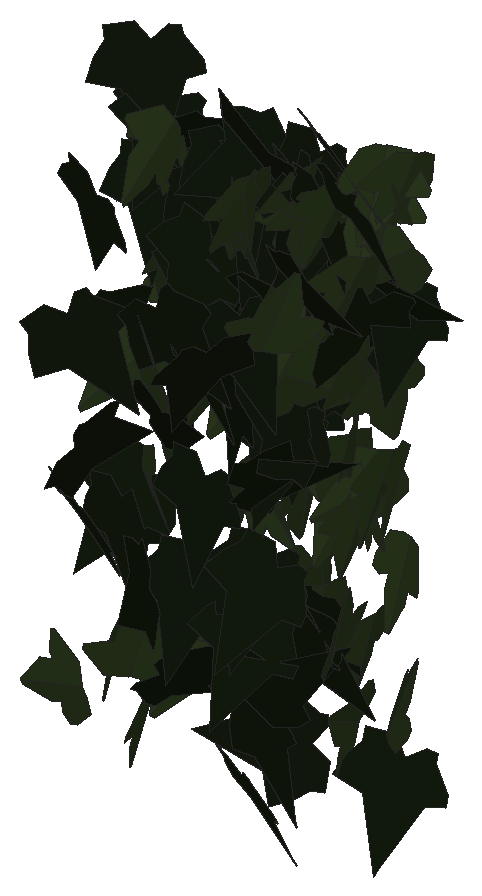
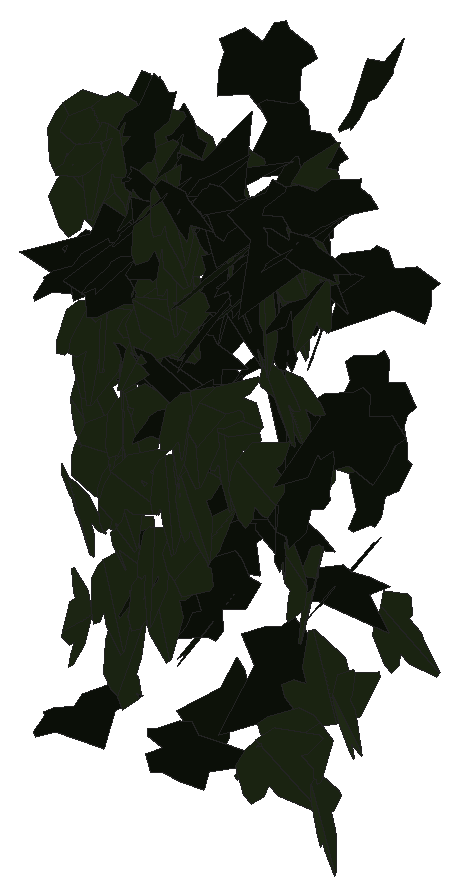
# SketchUp Ruby script. Lengths in inches.
U = 1.inch
M = Sketchup.active_model
def pt(a) = Geom::Point3d.new(a.map { |v| v * U })
def face(e, loops, mat)
  f = e.add_face(loops[0].map { |a| pt(a) })
  loops[1..].each { |l| e.add_face(l.map { |a| pt(a) }).erase! }
  f.material = f.back_material = mat if mat
  f
end
# faces: each face lists its corners as indices into pts; further lists are holes
def faces(e, pts, list, mat = nil) = list.each { |f| face(e, (f[0].is_a?(Array) ? f : [f]).map { |l| l.map { |i| pts[i] } }, mat) }
# xy, xz, yz: faces in a plane at the given z, y or x. An outline is a flat list of corners, or four numbers for a rectangle; further outlines are holes
def ring(l) = l.size == 4 ? [[l[0], l[1]], [l[2], l[1]], [l[2], l[3]], [l[0], l[3]]] : l.each_slice(2).to_a
def flat(e, list, mat, &to3) = list.each { |f| face(e, (f[0].is_a?(Array) ? f : [f]).map { |l| ring(l).map { |u, v| to3.(u, v) } }, mat) }
def xy(e, z, list, mat = nil) = flat(e, list, mat) { |x, y| [x, y, z] }
def xz(e, y, list, mat = nil) = flat(e, list, mat) { |x, z| [x, y, z] }
def yz(e, x, list, mat = nil) = flat(e, list, mat) { |y, z| [x, y, z] }
def lines(e, pts, list) = list.each { |a, b| e.add_line(pt(pts[a]), pt(pts[b])) }
# prism: a flat outline (further loops are holes) pulled along v
def prism(e, loops, v, mat = nil)
  f = face(e, loops, mat); d = Geom::Vector3d.new(v.map { |x| x * U })
  f.pushpull(f.normal.samedirection?(d) ? d.length : -d.length)
end
def box(e, o, s, mat = nil) = prism(e, [[o, [o[0] + s[0], o[1], o[2]], [o[0] + s[0], o[1] + s[1], o[2]], [o[0], o[1] + s[1], o[2]]]], [0, 0, s[2]], mat)
def at(x, y, z, deg = 0) = Geom::Transformation.translation(pt([x, y, z])) * Geom::Transformation.rotation(ORIGIN, Z_AXIS, deg.degrees)
def axes(o, x, y, z) = Geom::Transformation.new([*x, 0, *y, 0, *z, 0, *pt(o).to_a, 1])
def part(name) = M.definitions.add(name)
# library, detail: a bought-in or finely detailed component or shape, given as its bounding box
def library(name, o, s) = part(name).tap { |d| box(d.entities, o, s) }
def detail(e, o, s) = box(e.add_group.entities, o, s)
def put(e, d, t, mat = nil) = e.add_instance(d, t).tap { |i| i.material = mat if mat }
def group(e, t, mat = nil) = e.add_group.tap { |g| g.transformation = t; g.material = mat if mat }.entities
root = M.entities
M.materials.add("efeu1").color = [18, 25, 13]
M.materials.add("efeu2").color = [43, 57, 29]
c1 = part("ivyleaf_9")
p = [[1.54,2.16,1.25],[1.36,2.04,1.19],[-0.21,0.99,0.68],[-0.71,1.11,0.82],[-0.85,0.86,0.67],[-0.8,0.17,0.21],
  [-0.9,-0.01,0.1],[-0.67,-0.16,-0.02],[-0.08,-0.08,-0.05],[-0.03,-0.6,-0.4],[0.65,-0.88,-0.66],[0.83,-0.6,-0.49],
  [1.29,-0.42,-0.43],[1.8125,-0.07,-0.26],[1.21,0.44,0.15]]
faces(c1.entities,p,[[0,1,2,3,4,5,6,7,8,9,10,11,12,13,14]],"efeu1")
c2 = part("ivyleaf_10")
p = [[0,0.5,-0.03],[-0.0625,2.02,-0.43],[-0.19,2.01,-0.46],[-0.54,1.05,-0.29],[-0.52,0.625,-0.18],[-0.83,0.76,-0.28],
  [-1.16,0.64,-0.33],[-1.15,0.33,-0.24],[-0.77,-0.39,0.02],[-0.3,-0.51,0.16],[0.04,-0.48,0.23],[-0.02,2.01,-0.4375],
  [-0.06,2.01,-0.43],[0.04,-0.49,0.23],[0.67,-0.49,0.14],[1.38,0.36,-0.2],[1.375,0.51,-0.24],[0.81,0.65,-0.19],
  [0.62,0.59,-0.15],[0.6,1.09,-0.28],[0.5,1.23,-0.31]]
faces(c2.entities,p,[[0,1,2,3,4,5,6,7,8,9,10],[11,12,0,13,14,15,16,17,18,19,20]],"efeu2")
put(root,c1,axes([14.76,220.19,218.36],[0.00233,-0.19291,0.46128],[-0.0176,-0.46103,-0.19272],[0.49968,-0.01534,-0.00894]))
put(root,c1,axes([15.89,219.92,222.17],[-0.00179,0.43095,-0.25353],[0.00643,-0.25349,-0.43093],[-0.49996,-0.0048,-0.00464]))
put(root,c1,axes([13.15,221.18,222.89],[0.04405,-0.3663,0.33747],[0.11155,-0.32293,-0.36507],[0.4854,0.10745,0.05327]))
put(root,c2,axes([14.5,220.78,220.76],[-0.34497,0.29007,-0.21646],[-0.16391,0.1414,0.45071],[0.32269,0.38192,-0.00247]))
put(root,c1,axes([14.4,220.875,221.83],[-0.09481,-0.07375,-0.48536],[0.36921,0.31509,-0.12],[0.32356,-0.38115,-0.00529]))
put(root,c1,axes([14.35,221.52,221.02],[0.26151,-0.37801,0.19676],[0.11597,-0.15902,-0.45963],[0.41008,0.28604,0.0045]))
put(root,c1,axes([14.35,221.82,219.04],[0.01013,-0.48128,0.13516],[-0.00187,-0.13522,-0.48136],[0.49989,0.00925,-0.00454]))
put(root,c2,axes([12.44,221.62,215.58],[-0.14932,0.01669,0.47689],[-0.47701,-0.01868,-0.1487],[0.01285,-0.49937,0.0215]))
put(root,c1,axes([12.4375,221.58,220.76],[-0.09135,-0.19879,-0.4496],[0.23418,0.38447,-0.21758],[0.43222,-0.25032,0.02286]))
put(root,c1,axes([12.17,222.09,217.77],[0.16583,-0.32378,0.34303],[0.21202,-0.27364,-0.36079],[0.42136,0.26512,0.04654]))
put(root,c1,axes([12.59,221.54,219],[-0.07644,0.14771,-0.47153],[-0.19172,0.43089,0.16606],[0.45541,0.20619,-0.00924]))
put(root,c2,axes([15.23,222.02,221.27],[-0.25308,-0.41816,0.10533],[0.05625,0.08908,0.48877],[-0.42753,0.25925,0.00196]))
put(root,c1,axes([14.42,222.37,220.21],[0.08327,-0.02464,-0.4924],[0.43034,-0.24004,0.08479],[-0.24057,-0.43792,-0.01877]))
put(root,c1,axes([14.51,222.33,221.12],[-0.21539,-0.16792,-0.41882],[0.34983,0.23098,-0.27252],[0.285,-0.41043,0.01799]))
put(root,c1,axes([13.58,222.6,217.17],[-0.40393,-0.20462,-0.21206],[0.18625,0.10157,-0.45276],[0.22837,-0.44476,-0.00583]))
put(root,c1,axes([15.15,222.61,221.72],[0.2156,-0.21581,0.39616],[0.29563,-0.26407,-0.30475],[0.34076,0.36564,0.01373]))
put(root,c1,axes([14.42,222.82,216.58],[-0.25436,-0.42657,0.05779],[-0.03097,-0.04881,-0.49665],[0.42935,-0.25623,-0.00159]))
put(root,c1,axes([14.75,222.21,218.92],[0.24331,0.15965,0.40658],[0.32572,0.24378,-0.29065],[-0.29104,0.4063,0.01462]))
put(root,c1,axes([14.49,222.69,215.39],[0.23415,-0.44171,-0.00808],[-0.00222,0.00797,-0.49993],[0.44178,0.23415,0.00177]))
put(root,c1,axes([14.64,222.82,217.42],[-0.44396,-0.2181,-0.07301],[0.0657,0.03184,-0.49464],[0.22041,-0.4488,0.00038]))
put(root,c1,axes([15.05,222.9,219.41],[-0.07435,-0.49344,-0.03144],[0.00638,-0.03275,0.49889],[-0.4944,0.07378,0.01116]))
put(root,c1,axes([13.99,222.77,220.64],[-0.37748,0.25966,-0.20021],[0.17062,-0.10515,-0.45807],[-0.27999,-0.41415,-0.00923]))
put(root,c1,axes([13.42,223.08,221.42],[-0.14394,-0.43698,0.19579],[-0.04655,-0.1907,-0.45985],[0.47657,-0.15061,0.01422]))
put(root,c1,axes([14.4,222.97,217.41],[-0.40011,-0.25057,-0.1647],[0.14543,0.07801,-0.47198],[0.26223,-0.42559,0.01046]))
put(root,c1,axes([14.02,223.01,214.19],[0.2735,-0.33815,0.24669],[0.16205,-0.18616,-0.43484],[0.38593,0.31781,0.00776]))
put(root,c2,axes([12.6,223.19,222.66],[-0.06892,-0.23857,0.43397],[0.1444,-0.4288,-0.2128],[0.47371,0.096,0.128]))
put(root,c1,axes([13.52,223.17,220.99],[-0.33487,-0.32523,0.17912],[-0.12463,-0.12876,-0.46678],[0.34976,-0.35727,0.00517]))
put(root,c1,axes([14.76,223.02,219.53],[-0.40706,-0.24319,-0.15861],[0.13589,0.0818,-0.47417],[0.25658,-0.42915,-0.0005]))
put(root,c1,axes([14.4375,222.68,215.56],[0.01136,-0.04076,0.49821],[0.49281,0.08437,-0.00434],[-0.08371,0.49114,0.04209]))
put(root,c2,axes([14.11,222.86,222.42],[0.04549,-0.46584,-0.17584],[0.02049,0.17818,-0.46673],[0.49751,0.03526,0.0353]))
put(root,c1,axes([12.5,223.13,218.72],[0.39075,-0.02887,-0.31062],[0.31195,0.03349,0.38931],[-0.00167,-0.49804,0.04419]))
put(root,c2,axes([14.14,223.13,218.25],[0.11645,-0.04061,0.48455],[0.47413,-0.10105,-0.12241],[0.10787,0.488,0.01497]))
put(root,c2,axes([13.97,223.16,222.42],[-0.00729,-0.49591,0.06341],[0.01273,-0.06358,-0.49578],[0.49978,-0.00561,0.01356]))
put(root,c1,axes([11.84,223.35,217.19],[0.11225,-0.47964,0.08568],[0.02216,-0.08281,-0.4926],[0.48673,0.11439,0.00267]))
put(root,c2,axes([12.2,223.14,215.12],[-0.35819,-0.33698,0.09024],[0.06513,0.06246,0.49179],[-0.34272,0.36407,-0.00085]))
put(root,c2,axes([14.93,222.85,220.26],[-0.07034,-0.29149,-0.40011],[0.11045,0.3847,-0.29968],[0.48255,-0.13054,0.01027]))
put(root,c2,axes([15.31,223.25,216.375],[0.12151,-0.46907,-0.12331],[0.03017,-0.11957,0.48455],[-0.48407,-0.1252,-0.00076]))
put(root,c2,axes([13.95,223.12,218.52],[0.04535,-0.48928,-0.09248],[-0.01019,0.09193,-0.49137],[0.49783,0.04645,-0.00164]))
put(root,c1,axes([13.625,223.11,221.03],[0.2502,0.23742,-0.36199],[-0.24992,-0.26217,-0.34469],[-0.35347,0.35341,-0.01252]))
put(root,c2,axes([15.48,223.38,221.68],[-0.06555,-0.45576,0.19489],[-0.03657,-0.19161,-0.46038],[0.49433,-0.07461,-0.00821]))
put(root,c2,axes([15.1875,223.38,222.625],[-0.04592,-0.4622,0.18511],[-0.02941,-0.18305,-0.46436],[0.49702,-0.05353,-0.01038]))
put(root,c1,axes([12.88,222.86,215.33],[0.31253,0.31756,0.22689],[0.15886,0.162,-0.44555],[-0.3565,0.35058,0.00037]))
put(root,c2,axes([11.94,223.59,219.21],[-0.16176,-0.17978,0.43762],[-0.04447,-0.45467,-0.20322],[0.47102,-0.10466,0.1311]))
put(root,c2,axes([13.96,223.02,221.93],[-0.29436,0.18357,0.36008],[-0.3023,0.19568,-0.34688],[-0.26827,-0.42192,-0.00422]))
put(root,c1,axes([15.27,223.36,222.82],[0.32696,-0.36554,0.09736],[0.07151,-0.06665,-0.49035],[0.37146,0.33457,0.00869]))
put(root,c2,axes([12.68,223.37,221.24],[0.10919,-0.48776,0.01289],[-0.00313,-0.01391,-0.4998],[0.48792,0.10906,-0.00609]))
put(root,c2,axes([14.21,223.67,216.7],[-0.07187,-0.19121,-0.45637],[-0.14958,-0.43119,0.20422],[-0.47166,0.16588,0.00477]))
put(root,c2,axes([11.7,223.53,215.41],[0.25733,-0.35688,0.23752],[0.13949,-0.19225,-0.43998],[0.40537,0.2927,0.00062]))
put(root,c1,axes([14.61,223.41,216.32],[-0.00879,-0.00758,-0.49987],[0.4487,0.22033,-0.01123],[0.22044,-0.44877,0.00293]))
put(root,c2,axes([14.62,223.69,220.8],[-0.1549,-0.36837,0.30051],[0.03263,-0.32356,-0.3798],[0.47428,-0.09805,0.12428]))
put(root,c2,axes([14.75,223.53,222.34],[-0.0955,-0.48763,0.05562],[-0.01417,-0.0539,-0.49688],[0.49059,-0.09648,-0.00352]))
put(root,c1,axes([13.74,223.88,222.46],[-0.26539,-0.20554,0.37057],[-0.19383,-0.32995,-0.32182],[0.37683,-0.31447,0.09545]))
put(root,c1,axes([15.48,223.64,221.08],[0.0128,0.27704,-0.41604],[0.00528,-0.41623,-0.277],[-0.49981,0.00269,-0.01358]))
put(root,c1,axes([11.85,223.77,217.34],[-0.42796,-0.25826,0.0123],[-0.01042,-0.00653,-0.49985],[0.25835,-0.42809,0.00021]))
put(root,c2,axes([15.625,223.74,218.8125],[0.10429,-0.43982,0.21374],[0.09454,-0.19628,-0.45004],[0.47978,0.13428,0.04223]))
put(root,c1,axes([14.61,223.84,222.2],[0.1447,-0.42618,0.21779],[0.09806,-0.1963,-0.44928],[0.46845,0.17273,0.02677]))
put(root,c2,axes([13.5,223.94,219.36],[-0.19559,-0.2325,0.3971],[0.03401,-0.43761,-0.23947],[0.4589,-0.06667,0.187]))
put(root,c2,axes([14.52,223.875,220.44],[-0.20464,-0.34136,0.30264],[-0.05573,-0.3105,-0.38792],[0.45279,-0.19251,0.08903]))
put(root,c1,axes([11.5,223.3125,219.65],[-0.00963,0.02581,-0.49924],[0.00755,0.49928,0.02567],[0.49985,-0.00704,-0.01001]))
put(root,c2,axes([14.98,224.03,214.9],[-0.0206,-0.23162,-0.44264],[0.02009,-0.44304,0.23089],[-0.49917,-0.00828,0.02756]))
put(root,c1,axes([12.0625,224.05,222.34],[-0.15806,-0.43301,0.19371],[0.02874,-0.21254,-0.45166],[0.47349,-0.13164,0.09208]))
put(root,c1,axes([14.625,223.82,223.03],[0.32369,-0.30838,0.22389],[0.16021,-0.15642,-0.44706],[0.34578,0.36115,-0.00245]))
put(root,c1,axes([13.67,223.82,222.22],[0.35782,-0.20261,0.28446],[-0.23855,0.15564,0.41094],[-0.25506,-0.4298,0.01472]))
put(root,c2,axes([14.31,223.68,221.23],[0.02098,-0.48878,-0.10322],[0.02264,0.10414,-0.48851],[0.49905,0.01582,0.0265]))
put(root,c1,axes([12.8,223.81,221.78],[0.08015,-0.47079,-0.14808],[-0.00513,0.14922,-0.47719],[0.49351,0.07801,0.01909]))
put(root,c1,axes([14.79,223.97,216.13],[0.20306,-0.45665,0.01539],[-0.00616,0.01411,0.49976],[-0.45687,-0.20316,0.00011]))
put(root,c1,axes([13.53,224.1,221.29],[-0.10276,-0.41799,0.25441],[0.07404,-0.27025,-0.41411],[0.48369,-0.04743,0.11743]))
put(root,c1,axes([12.31,223.99,217.69],[0.01794,0.12826,0.48294],[-0.03302,-0.48189,0.12921],[0.49859,-0.03653,-0.00882]))
put(root,c1,axes([13.24,223.82,222.46],[-0.25159,-0.26687,-0.33983],[0.2496,0.23123,-0.36638],[0.3527,-0.354,0.01687]))
put(root,c2,axes([15.36,223.61,220.3],[-0.0429,-0.43668,-0.23973],[0.02218,0.23871,-0.43878],[0.49766,-0.04828,-0.00111]))
put(root,c1,axes([11.91,223.99,221.6],[-0.05686,-0.4967,-0.00739],[-0.00192,0.00765,-0.49994],[0.49675,-0.05682,-0.00278]))
put(root,c2,axes([15.53,223.85,222.98],[0.24271,0.40499,-0.16455],[-0.09269,-0.13626,-0.47206],[-0.4272,0.25965,0.00894]))
put(root,c2,axes([15.8,223.87,221.85],[-0.26663,-0.15035,0.39535],[-0.35102,-0.18211,-0.30598],[0.236,-0.44072,-0.00844]))
put(root,c2,axes([14.93,223.87,218.8],[-0.07713,-0.48882,0.07145],[-0.00115,-0.07213,-0.49477],[0.49401,-0.07648,0.01001]))
put(root,c1,axes([12.27,224.01,220.66],[-0.01992,0.07124,0.4945],[0.16452,-0.46635,0.07382],[0.47174,0.16565,-0.00486]))
put(root,c1,axes([14.06,224.03,219.24],[-0.05955,-0.49592,-0.02268],[-0.00064,0.02292,-0.49947],[0.49644,-0.05946,-0.00336]))
put(root,c2,axes([15.625,224.07,218.72],[0.19324,-0.34034,0.31116],[0.18527,-0.25165,-0.39031],[0.42229,0.26615,0.02885]))
put(root,c2,axes([14.24,223.9,222.32],[-0.00719,-0.49907,0.02962],[-0.00172,-0.0296,-0.49912],[0.49995,-0.00728,-0.00129]))
put(root,c2,axes([12.59,223.875,220.1875],[0.42068,-0.26124,-0.06914],[-0.05887,0.03626,-0.4952],[0.26374,0.42478,-0.00025]))
put(root,c2,axes([12.37,223.875,220.13],[0.48329,-0.10835,-0.06849],[-0.06572,0.01993,-0.49526],[0.11005,0.48771,0.00503]))
put(root,c2,axes([14.31,223.96,221.92],[-0.23436,-0.41396,0.15399],[-0.03715,-0.15523,-0.47384],[0.44011,-0.23353,0.042]))
put(root,c1,axes([14.55,223.61,221.23],[-0.11844,-0.19119,0.44656],[0.27559,0.35207,0.22382],[-0.40003,0.29916,0.02199]))
put(root,c2,axes([12.05,223.66,217.44],[-0.33351,0.32474,0.18254],[-0.12767,0.13052,-0.46547],[-0.34996,-0.35708,-0.00414]))
put(root,c2,axes([14.64,223.65,220.16],[-0.19237,-0.34336,-0.30838],[0.13351,0.2784,-0.39328],[0.44178,-0.23366,-0.01543]))
put(root,c1,axes([12.69,224.23,221.51],[-0.09727,-0.40747,0.27296],[0.0538,-0.28547,-0.40696],[0.48749,-0.0498,0.09938]))
put(root,c2,axes([11.77,223.92,214.14],[0.21207,-0.45278,-0.00373],[-0.00118,0.00356,-0.49999],[0.4528,0.21207,0.00045]))
put(root,c2,axes([15.33,223.9,222.52],[0.37016,0.32502,-0.08565],[-0.06224,-0.05893,-0.4926],[-0.33031,0.37535,-0.00317]))
put(root,c1,axes([14.41,224.21,222.07],[-0.07144,-0.45532,0.19385],[0.02018,-0.19838,-0.45852],[0.49446,-0.05769,0.04672]))
put(root,c2,axes([15.76,224.06,222.93],[-0.08003,-0.46234,0.17274],[0.01401,-0.17705,-0.46739],[0.49336,-0.06997,0.04129]))
put(root,c2,axes([12.09,223.85,222.2],[0.47843,-0.11636,-0.08697],[-0.05503,0.13186,-0.47915],[0.13444,0.46805,0.11336]))
put(root,c2,axes([15.04,224.125,218.0625],[0.02269,-0.08425,0.49233],[0.44609,-0.21829,-0.05792],[0.2247,0.44187,0.06526]))
put(root,c2,axes([15.08,223.83,219.17],[0.22622,-0.41478,-0.16366],[-0.0058,0.18076,-0.46615],[0.44586,0.2128,0.07697]))
put(root,c2,axes([14.78,224.22,217.97],[-0.13281,-0.32268,0.35811],[0.08012,-0.38106,-0.31365],[0.47533,-0.02593,0.15292]))
put(root,c2,axes([14.27,223.91,218.1],[0.04048,-0.48946,-0.09376],[-0.00827,0.09339,-0.49113],[0.49829,0.04131,-0.00054]))
put(root,c2,axes([14.42,224,216.44],[-0.09228,-0.48988,0.03881],[-0.00941,-0.03772,-0.49849],[0.49132,-0.09273,-0.00226]))
put(root,c1,axes([12.35,223.64,222.43],[0.33984,0.36401,0.04483],[0.03329,0.03025,-0.49797],[-0.36524,0.34144,-0.00368]))
put(root,c2,axes([15.18,224,216.29],[0.02651,-0.49907,0.0151],[0.00274,-0.01498,-0.49977],[0.49929,0.02659,0.00194]))
put(root,c2,axes([15.23,224.25,218.3],[-0.06505,-0.18947,0.45811],[-0.16765,-0.42641,-0.20017],[0.46654,-0.17965,-0.00806]))
put(root,c1,axes([14.11,224.14,214.22],[-0.18609,-0.23176,-0.40207],[-0.26787,-0.3001,0.29696],[-0.37897,0.32593,-0.01247]))
put(root,c2,axes([15.6,223.91,219.96],[-0.13232,-0.47278,-0.09471],[0.02416,0.09158,-0.49095],[0.48157,-0.1345,-0.00139]))
put(root,c1,axes([14.6,224.1,219.8],[-0.49059,-0.03524,-0.08991],[0.08958,0.00785,-0.49185],[0.03608,-0.49869,-0.00139]))
put(root,c2,axes([13.8,224.07,218.07],[0.12887,-0.47892,0.06346],[0.00601,-0.06409,-0.49584],[0.48307,0.12856,-0.01076]))
put(root,c1,axes([11.7,224.07,223.26],[-0.17582,-0.41218,-0.2218],[0.07618,0.20857,-0.44799],[0.46182,-0.19133,-0.01054]))
put(root,c1,axes([14.81,224.04,221.21],[0.10351,-0.463,-0.15784],[0.005,0.16233,-0.47289],[0.48914,0.09632,0.03823]))
put(root,c1,axes([13.39,224.04,220.86],[0.22089,-0.43785,-0.09746],[-0.04558,0.08616,-0.49041],[0.44624,0.22554,-0.00185]))
put(root,c2,axes([15.67,224.07,217.45],[0.44015,-0.23276,0.04577],[0.03963,-0.02296,-0.4979],[0.23388,0.44192,-0.00176]))
put(root,c2,axes([14.24,223.68,220.22],[0.19104,0.26655,-0.37743],[0.19742,0.32217,0.32746],[0.41776,-0.27414,0.01785]))
put(root,c2,axes([12.67,223.88,221.3125],[0.13428,-0.41855,-0.23829],[-0.06612,0.22901,-0.43952],[0.47707,0.14955,0.00615]))
put(root,c2,axes([11.9,223.92,221.73],[-0.46472,0.18177,-0.03146],[0.03453,0.00194,-0.4988],[-0.18121,-0.46578,-0.01435]))
put(root,c2,axes([14.9375,224.16,217.875],[0.02085,-0.48689,0.11181],[0.02591,-0.1107,-0.4869],[0.49889,0.0261,0.02062]))
put(root,c1,axes([15.51,224.28,214.4],[-0.20191,-0.45709,-0.01743],[0.0052,0.01676,-0.49969],[0.45739,-0.20197,-0.00201]))
put(root,c2,axes([15.86,223.72,215.35],[0.11342,-0.13923,0.46664],[-0.27896,0.37415,0.17943],[-0.39915,-0.30105,0.00719]))
put(root,c2,axes([15.375,223.93,222.67],[-0.47108,0.14417,0.08543],[-0.07718,0.03962,-0.49242],[-0.14875,-0.47712,-0.01507]))
put(root,c1,axes([15.52,224.32,220.96],[-0.10949,-0.48663,0.03471],[-0.00313,-0.03488,-0.49877],[0.48786,-0.10943,0.0046]))
put(root,c2,axes([13.8,224.28,218.59],[-0.12731,0.03892,0.48195],[0.41834,-0.24105,0.12997],[0.24246,0.43633,0.02881]))
put(root,c1,axes([14.23,224.2,222.51],[-0.41419,-0.13719,-0.24418],[0.22969,0.08308,-0.43628],[0.16028,-0.47358,-0.0058]))
put(root,c2,axes([14.45,223.95,217],[0.03921,-0.45295,-0.20807],[-0.00947,0.208,-0.45458],[0.49837,0.03959,0.00773]))
put(root,c1,axes([11.96,224.23,222.51],[-0.47284,-0.11375,-0.1161],[0.11257,0.02844,-0.48633],[0.11725,-0.48606,-0.00128]))
put(root,c2,axes([15.26,223.97,219.99],[-0.17108,-0.43764,-0.17088],[0.05904,0.16039,-0.46988],[0.4661,-0.18095,-0.0032]))
put(root,c2,axes([12.32,224.3,214.81],[-0.25894,-0.28692,0.31721],[-0.11941,-0.30758,-0.37568],[0.41072,-0.27031,0.09077]))
put(root,c1,axes([11.64,224.29,218.76],[0.41245,-0.11927,-0.25624],[0.25627,-0.03337,0.42803],[-0.11921,-0.48442,0.0336]))
put(root,c2,axes([11.81,224.32,217.63],[-0.02227,0.0369,-0.49814],[0.32475,-0.3778,-0.0425],[-0.37953,-0.32543,-0.00714]))
put(root,c2,axes([13.71,224.11,219.35],[-0.17654,-0.46779,-0.00282],[0.00031,0.0029,-0.49999],[0.4678,-0.17654,-0.00073]))
put(root,c1,axes([14.96,224.02,220.96],[0.30332,-0.06669,0.39185],[0.38338,-0.08106,-0.31056],[0.10495,0.48886,0.00196]))
put(root,c2,axes([12.07,223.88,215.02],[-0.18594,-0.21061,-0.41361],[0.34127,0.23995,-0.2756],[0.31458,-0.38479,0.05452]))
put(root,c2,axes([12.58,224.34,218.91],[0.00231,-0.41776,0.27472],[-0.01312,-0.27468,-0.41759],[0.49982,-0.00528,-0.01224]))
